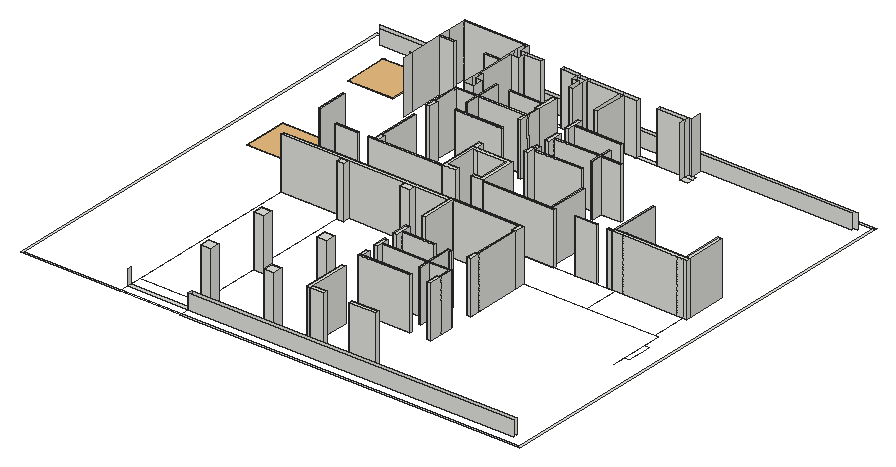
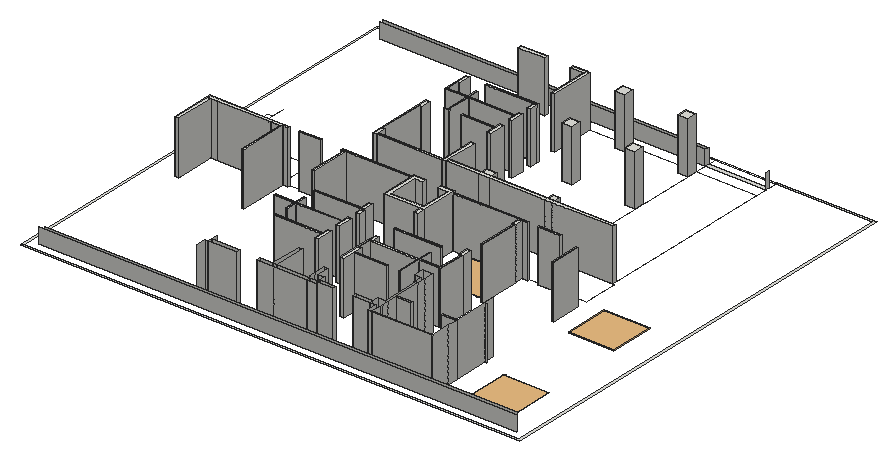
# SketchUp Ruby script. Lengths in inches.
U = 1.inch
M = Sketchup.active_model
def pt(a) = Geom::Point3d.new(a.map { |v| v * U })
def face(e, loops, mat)
  f = e.add_face(loops[0].map { |a| pt(a) })
  loops[1..].each { |l| e.add_face(l.map { |a| pt(a) }).erase! }
  f.material = f.back_material = mat if mat
  f
end
# faces: each face lists its corners as indices into pts; further lists are holes
def faces(e, pts, list, mat = nil) = list.each { |f| face(e, (f[0].is_a?(Array) ? f : [f]).map { |l| l.map { |i| pts[i] } }, mat) }
# xy, xz, yz: faces in a plane at the given z, y or x. An outline is a flat list of corners, or four numbers for a rectangle; further outlines are holes
def ring(l) = l.size == 4 ? [[l[0], l[1]], [l[2], l[1]], [l[2], l[3]], [l[0], l[3]]] : l.each_slice(2).to_a
def flat(e, list, mat, &to3) = list.each { |f| face(e, (f[0].is_a?(Array) ? f : [f]).map { |l| ring(l).map { |u, v| to3.(u, v) } }, mat) }
def xy(e, z, list, mat = nil) = flat(e, list, mat) { |x, y| [x, y, z] }
def xz(e, y, list, mat = nil) = flat(e, list, mat) { |x, z| [x, y, z] }
def yz(e, x, list, mat = nil) = flat(e, list, mat) { |y, z| [x, y, z] }
def lines(e, pts, list) = list.each { |a, b| e.add_line(pt(pts[a]), pt(pts[b])) }
# prism: a flat outline (further loops are holes) pulled along v
def prism(e, loops, v, mat = nil)
  f = face(e, loops, mat); d = Geom::Vector3d.new(v.map { |x| x * U })
  f.pushpull(f.normal.samedirection?(d) ? d.length : -d.length)
end
def box(e, o, s, mat = nil) = prism(e, [[o, [o[0] + s[0], o[1], o[2]], [o[0] + s[0], o[1] + s[1], o[2]], [o[0], o[1] + s[1], o[2]]]], [0, 0, s[2]], mat)
def at(x, y, z, deg = 0) = Geom::Transformation.translation(pt([x, y, z])) * Geom::Transformation.rotation(ORIGIN, Z_AXIS, deg.degrees)
def axes(o, x, y, z) = Geom::Transformation.new([*x, 0, *y, 0, *z, 0, *pt(o).to_a, 1])
def part(name) = M.definitions.add(name)
# library, detail: a bought-in or finely detailed component or shape, given as its bounding box
def library(name, o, s) = part(name).tap { |d| box(d.entities, o, s) }
def detail(e, o, s) = box(e.add_group.entities, o, s)
def put(e, d, t, mat = nil) = e.add_instance(d, t).tap { |i| i.material = mat if mat }
def group(e, t, mat = nil) = e.add_group.tap { |g| g.transformation = t; g.material = mat if mat }.entities
root = M.entities
c1 = library("BED",[-54,-53,-0.5],[108,106,1])
c2 = part("zw$FF1D")
put(c2.entities,c1,at(140.52,-153.67,0.04,-179.97))
put(c2.entities,c1,at(-181.99,-153.67,0.04,-179.97))
put(c2.entities,c1,at(-188.6,153.33,0.04,0.03))
box(root,[7152.21,596.5,1.375],[4.52,73.45,126])
box(root,[7210.71,572.45,1.375],[53.1,4.5,122.5625])
box(root,[7300.73,60,1.375],[24,24,122.5625])
box(root,[7300.73,217.5,1.375],[24,24,122.5625])
box(root,[7450.73,60,1.375],[24,24,122.5625])
box(root,[7450.73,217.5,1.375],[24,24,122.5625])
box(root,[7653.13,60,1.375],[63.82,9,122.5625])
xy(root,1.375,[[6920.46,0,7156.71,0,7156.71,4.5,6924.96,4.5,6924.96,1056.5,8106.96,1056.5,8106.96,1061,6920.46,1061],[7300.7,0,8102.46,4.5],[8102.46,0,8106.96,1056.5],[7156.71,24,7300.7,33],[7552.71,60,7561.71,165],
  [7561.71,60,7593.13,69],[7552.73,213,7676.4375,217.41],[7716.98,213,7725.96,241.45],[7552.73,217.41,7561.71,237],[7721.48,241.45,7725.96,271.5],
  [7669.71,247.5,7674.21,271.5],[7552.71,261,7561.71,292.1],[7561.71,271.5,7669.71,276],[7669.71,271.5,7674.21,276],[7674.21,271.5,7725.96,276],
  [7669.71,276,7674.21,331.02],[7552.71,316.1,7561.71,355],[7561.71,331,7638.96,335.5],[7716.98,331,7725.96,355],[7669.71,331.02,7674.21,331.5],
  [7674.21,331.02,7674.21,331.5,7669.71,331.5,7669.71,335.5,7680.96,335.5,7680.96,331.02],[7721.46,355,7725.96,464.5],[7552.7,403,7561.71,488.5],[7716.96,464.5,7725.98,488.5],[7300.71,464.55,7317.23,479.5],
  [7561.73,484.03,7716.96,488.5],[7450.73,488.5,7474.73,488.55],[7287.8125,572.5,7465.71,576.95],[7465.71,572.5,7465.71,662.5,7561.71,662.5,7561.71,572.5,7534.71,572.5,7534.71,581.5,7552.71,581.5,7552.71,653.5,7474.71,653.5,7474.71,581.5,7498.71,581.5,7498.71,572.5],[7561.71,572.5,7731.96,577],
  [7300.71,576.95,7309.73,596.85],[7719.96,577,7725.9375,670],[7300.71,596.85,7305.21,693.9375],[7465.71,662.5,7474.73,681.95],[7552.71,706,7561.71,730],
  [7561.71,725.5,7674.1875,730],[7300.73,730,7309.71,754],[7552.71,730,7561.71,745.14],[7353.21,749.45,7465.71,753.92],[7300.71,754,7305.23,818.45],
  [7669.71,760,7674.21,813.5],[7552.71,769.14,7561.71,804.6],[7561.71,784,7669.71,788.5],[7674.21,784,7721.46,788.5],[7465.71,795.95,7474.71,813.95],
  [7305.23,813.95,7353.21,818.45],[7357.71,813.95,7474.71,818.45],[7552.71,828.6,7561.71,867.45],[7300.71,843.5,7324.76,843.5,7324.76,867.5,7309.71,867.5,7309.71,886.95,7305.21,886.95,7305.21,977,7324.76,977,7324.76,1001,7309.7,1001,7309.7,1024.95,7300.71,1024.95,7300.71,952.95,7264.14,952.95,7264.14,948.45,7300.71,948.45],[7561.71,843.5,7674.1875,848],
  [7465.71,848,7474.71,900.43],[7552.71,915.5,7561.73,991.95],[7156.71,948.45,7193.27,952.95],[7708.01,977,7725.98,1001],[7324.76,991.95,7363.71,992],
  [7474.71,991.95,7552.71,992],[7552.71,991.95,7561.73,992],[7561.73,991.95,7592.49,992],[7324.76,992,7363.71,1001],[7450.7,992,7474.71,1001],
  [7474.71,992,7592.49,1001],[7592.49,992,7640.49,1001],[7640.49,992,7708.01,1001],[7411.71,1001,7450.7,1001.04],[7640.49,1001,7708.01,1001.04],
  [7156.71,1022.95,7300.71,1024.95]])
xy(root,4.8125,[[7552.71,706,7561.71,730]])
xy(root,123.9375,[[7552.71,60,7561.71,165],[7561.71,60,7593.13,69],[7552.73,213,7676.4375,217.41],[7716.98,213,7725.96,241.45],[7552.73,217.41,7561.71,237],
  [7721.48,241.45,7725.96,271.5],[7669.71,247.5,7674.21,271.5],[7552.71,261,7561.71,292.1],[7561.71,271.5,7669.71,276],[7669.71,271.5,7674.21,276],
  [7674.21,271.5,7725.96,276],[7669.71,276,7674.21,331.02],[7552.71,316.1,7561.71,355],[7561.71,331,7638.96,335.5],[7716.98,331,7725.96,355],
  [7674.21,331.02,7680.96,331.02,7680.96,335.5,7669.71,335.5,7669.71,331.5,7674.21,331.5],[7721.46,355,7725.96,464.5],[7552.7,403,7561.71,488.5],[7450.73,464.5,7474.73,479.5],[7716.96,464.5,7725.98,488.5],
  [7300.71,464.55,7317.23,479.5],[7156.71,479.5,7300.71,488.5],[7300.71,479.5,7317.23,488.5],[7317.23,479.5,7450.73,488.5],[7450.73,479.5,7474.73,488.5],
  [7474.73,479.5,7552.7,488.5],[7561.73,484.03,7716.96,488.5],[7287.8125,572.5,7465.71,576.95],[7561.71,572.5,7731.96,577],[7300.71,576.95,7309.73,596.85],
  [7719.96,577,7725.9375,670],[7300.71,596.85,7305.21,693.9375],[7561.71,725.5,7674.1875,730],[7552.71,730,7561.71,745.14],[7669.71,760,7674.21,813.5],
  [7552.71,769.14,7561.71,804.6],[7561.71,784,7669.71,788.5],[7674.21,784,7721.46,788.5],[7552.71,828.6,7561.71,867.45],[7561.71,843.5,7674.1875,848]])
xy(root,126,[[7353.21,749.45,7465.71,753.92]])
xy(root,127.375,[[7465.71,572.5,7498.71,572.5,7498.71,581.5,7474.71,581.5,7474.71,653.5,7552.71,653.5,7552.71,581.5,7534.71,581.5,7534.71,572.5,7561.71,572.5,7561.71,662.5,7465.71,662.5],[7465.71,662.5,7474.73,681.95],[7552.71,706,7561.71,730],[7300.73,730,7309.71,754],[7353.21,749.45,7465.71,753.92],
  [7300.71,754,7305.23,818.45],[7353.21,783.95,7357.71,871.95],[7465.71,795.95,7474.7,813.95],[7305.23,813.95,7353.21,818.45],[7357.71,813.95,7474.7,813.95,7474.71,818.45,7357.71,818.45],
  [7470.21,818.45,7474.71,847.95],[7465.71,848,7474.71,900.43],[7387.71,867.45,7465.71,871.95]])
xz(root,24,[[7300.7,1.375,8073.98,37.375]])
xz(root,33,[[7300.7,1.375,8073.98,37.375]])
xz(root,60,[[7552.71,1.375,7561.71,123.9375],[7561.71,1.375,7593.13,123.9375]])
xz(root,69,[[7561.71,1.375,7593.13,123.9375]])
xz(root,165,[[7552.71,1.375,7561.71,123.9375]])
xz(root,213,[[7552.73,1.375,7676.4375,123.9375],[7716.98,1.375,7725.96,123.9375]])
xz(root,217.41,[[7552.73,1.375,7561.71,123.9375],[7561.71,1.375,7676.4375,123.9375]])
xz(root,237,[[7552.73,1.375,7561.71,123.9375]])
xz(root,241.45,[[7716.98,1.375,7721.48,123.9375],[7721.48,1.375,7725.96,123.9375]])
xz(root,247.5,[[7669.71,1.375,7674.21,123.9375]])
xz(root,261,[[7552.71,1.375,7561.71,123.9375]])
xz(root,271.5,[[7561.71,1.375,7669.71,123.9375],[7669.71,1.375,7674.21,123.9375],[7674.21,1.375,7721.48,123.9375],[7721.48,1.375,7725.96,123.9375]])
xz(root,276,[[7561.71,1.375,7669.71,123.9375],[7669.71,1.375,7674.21,123.9375],[7674.21,1.375,7725.96,123.9375]])
xz(root,292.1,[[7552.71,1.375,7561.71,123.9375]])
xz(root,316.1,[[7552.71,1.375,7561.71,123.9375]])
xz(root,331,[[7561.71,1.375,7638.96,123.9375],[7716.98,1.375,7725.96,123.9375]])
xz(root,331.02,[[7669.71,1.375,7674.21,123.9375],[7674.21,1.375,7680.96,123.9375]])
xz(root,331.5,[[7669.71,1.375,7674.21,123.9375]])
xz(root,335.5,[[7561.71,1.375,7638.96,123.9375],[7669.71,1.375,7680.96,123.9375]])
xz(root,355,[[7552.71,1.375,7561.71,123.9375],[7716.98,1.375,7721.46,123.9375],[7721.46,1.375,7725.96,123.9375]])
xz(root,403,[[7552.7,1.375,7561.71,123.9375]])
xz(root,464.5,[[7450.73,1.375,7474.73,123.9375],[7716.96,1.375,7721.46,123.9375],[7721.46,1.375,7725.96,123.9375],[7725.96,1.375,7725.98,123.9375]])
xz(root,464.55,[[7300.71,1.375,7317.23,123.9375]])
xz(root,479.5,[[7156.71,1.375,7300.71,123.9375],[7300.71,1.375,7317.23,123.9375],[7317.23,1.375,7450.73,123.9375],[7474.73,1.375,7552.7,123.9375]])
xz(root,484.03,[[7561.73,1.375,7716.96,123.9375]])
xz(root,488.5,[[7156.71,1.375,7300.71,123.9375],[7300.71,1.375,7317.23,123.9375],[7317.23,1.375,7450.73,123.9375],[7450.73,1.375,7474.73,123.9375],[7474.73,1.375,7552.7,123.9375],
  [7552.7,1.375,7561.71,123.9375],[7561.73,1.375,7716.96,123.9375],[7716.96,1.375,7725.98,123.9375]])
xz(root,572.5,[[7287.8125,1.375,7465.71,123.9375],[7465.71,1.375,7498.71,127.375],[7534.71,1.375,7561.71,127.375],[7561.71,1.375,7731.96,123.9375]])
xz(root,576.95,[[7287.8125,1.375,7300.71,123.9375],[7300.71,1.375,7309.73,123.9375],[7309.73,1.375,7465.71,123.9375]])
xz(root,577,[[7561.71,1.375,7719.96,123.9375],[7719.96,1.375,7725.9375,123.9375],[7725.9375,1.375,7731.96,123.9375]])
xz(root,581.5,[[7474.71,1.375,7498.71,127.375],[7534.71,1.375,7552.71,127.375]])
xz(root,596.85,[[7300.71,1.375,7305.21,123.9375],[7305.21,1.375,7309.73,123.9375]])
xz(root,653.5,[[7474.71,1.375,7481.96,127.375],[7481.96,1.375,7545.45,127.375],[7545.45,1.375,7552.71,127.375]])
xz(root,662.5,[[7465.71,1.375,7474.73,127.375],[7474.73,1.375,7561.71,127.375]])
xz(root,670,[[7719.96,1.375,7725.9375,123.9375]])
xz(root,681.95,[[7465.71,1.375,7474.73,127.375]])
xz(root,693.9375,[[7300.71,1.375,7305.21,123.9375]])
xz(root,706,[[7552.71,1.375,7561.71,4.8125],[7552.71,4.8125,7561.71,127.375]])
xz(root,725.5,[[7561.71,1.375,7674.1875,123.9375]])
xz(root,730,[[7300.73,1.375,7309.71,127.375],[7552.71,1.375,7561.71,4.8125],[7561.71,1.375,7674.1875,123.9375],[7552.71,4.8125,7561.71,123.9375],[7552.71,123.9375,7561.71,127.375]])
xz(root,745.14,[[7552.71,1.375,7561.71,123.9375]])
xz(root,749.45,[[7353.21,1.375,7465.71,126],[7353.21,126,7465.71,127.375]])
xz(root,753.92,[[7353.21,1.375,7465.71,126],[7353.21,126,7465.71,127.375]])
xz(root,754,[[7300.71,1.375,7300.73,127.375],[7300.73,1.375,7305.23,127.375],[7305.23,1.375,7309.71,127.375]])
xz(root,760,[[7669.71,1.375,7674.21,123.9375]])
xz(root,769.14,[[7552.71,1.375,7561.71,123.9375]])
xz(root,783.95,[[7353.21,1.375,7357.71,127.375]])
xz(root,784,[[7561.71,1.375,7669.71,123.9375],[7674.21,1.375,7721.46,123.9375]])
xz(root,788.5,[[7561.71,1.375,7669.71,123.9375],[7674.21,1.375,7721.46,123.9375]])
xz(root,795.95,[[7465.71,1.375,7474.71,1.375,7474.7,127.375,7465.71,127.375]])
xz(root,804.6,[[7552.71,1.375,7561.71,123.9375]])
xz(root,813.5,[[7669.71,1.375,7674.21,123.9375]])
xz(root,813.95,[[7305.23,1.375,7353.21,127.375],[7357.71,1.375,7465.71,127.375],[7465.71,1.375,7465.71,127.375,7474.7,127.375,7474.71,1.375]])
xz(root,818.45,[[7300.71,1.375,7305.23,127.375],[7305.23,1.375,7353.21,127.375],[7357.71,1.375,7470.21,127.375],[7470.21,1.375,7474.71,127.375]])
xz(root,828.6,[[7552.71,1.375,7561.71,123.9375]])
xz(root,843.5,[[7300.71,1.375,7324.76,127.375],[7561.71,1.375,7674.1875,123.9375]])
xz(root,847.95,[[7470.21,1.375,7474.71,127.375]])
xz(root,848,[[7465.71,1.375,7474.71,127.375],[7561.71,1.375,7674.1875,123.9375]])
xz(root,867.45,[[7152.23,1.375,7156.71,127.375],[7387.71,1.375,7465.71,127.375],[7552.71,1.375,7561.71,123.9375]])
xz(root,867.5,[[7309.71,1.375,7324.76,127.375]])
xz(root,871.95,[[7353.21,1.375,7357.71,127.375],[7387.71,1.375,7465.71,127.375]])
xz(root,886.95,[[7305.21,1.375,7309.71,127.375]])
xz(root,900.43,[[7465.71,1.375,7474.71,127.375]])
xz(root,915.5,[[7552.71,1.375,7561.73,123.9375]])
xz(root,948.43,[[7465.71,1.375,7474.71,127.375]])
xz(root,948.45,[[7156.71,1.375,7193.27,127.375],[7264.14,1.375,7300.71,127.375]])
xz(root,952.95,[[7156.71,1.375,7193.27,127.375],[7264.14,1.375,7300.71,127.375]])
xz(root,976.95,[[7450.7,1.375,7465.71,127.375]])
xz(root,977,[[7305.21,1.375,7324.76,127.375]])
xz(root,991.95,[[7552.71,1.375,7561.73,123.9375]])
xz(root,992,[[7324.76,1.375,7363.71,127.375],[7411.71,1.375,7450.7,127.375],[7450.7,1.375,7474.71,123.9375],[7474.71,1.375,7552.71,123.9375],[7552.71,1.375,7561.73,123.9375],
  [7561.73,1.375,7592.49,123.9375],[7640.49,1.375,7708.01,123.9375]])
xz(root,1001,[[7309.7,1.375,7324.76,127.375],[7324.76,1.375,7363.71,127.375],[7411.71,1.375,7450.7,127.375],[7450.7,1.375,7474.71,123.9375],[7474.71,1.375,7552.71,123.9375],
  [7552.71,1.375,7592.49,123.9375],[7640.49,1.375,7708.01,123.9375],[7708.01,1.375,7716.96,123.9375]])
xz(root,1022.95,[[7156.71,1.375,7300.71,127.375]])
xz(root,1024.95,[[7156.71,1.375,7300.71,127.375],[7300.71,1.375,7309.7,127.375]])
xz(root,1028,[[6953.48,1.375,8073.98,37.375]])
xz(root,1037,[[6944.48,1.375,8082.98,37.375]])
yz(root,7156.71,[[24,1.375,33,37.375],[479.5,1.375,488.5,123.9375],[843.45,1.375,867.45,127.375],[867.45,1.375,948.45,127.375],[952.95,1.375,976.95,127.375],
  [976.95,1.375,1022.95,127.375],[1022.95,1.375,1024.95,127.375]])
yz(root,7193.27,[[948.45,1.375,952.95,127.375]])
yz(root,7264.14,[[948.45,1.375,952.95,127.375]])
yz(root,7287.8125,[[572.5,1.375,576.95,123.9375]])
yz(root,7300.7,[[24,1.375,33,37.375]])
yz(root,7300.71,[[464.55,1.375,479.5,123.9375],[576.95,1.375,596.85,123.9375],[596.85,1.375,693.9375,123.9375],[754,1.375,818.45,127.375],[843.5,1.375,867.5,127.375],
  [867.5,1.375,886.95,127.375],[886.95,1.375,948.45,127.375],[952.95,1.375,977,127.375],[977,1.375,992,127.375],[992,1.375,1001,127.375],
  [1001,1.375,1022.95,127.375],[1022.95,1.375,1024.95,127.375]])
yz(root,7300.73,[[730,1.375,754,127.375]])
yz(root,7305.21,[[596.85,1.375,693.9375,123.9375],[886.95,1.375,977,127.375]])
yz(root,7305.23,[[754,1.375,813.95,127.375],[813.95,1.375,818.45,127.375]])
yz(root,7309.7,[[1001,1.375,1024.95,127.375]])
yz(root,7309.71,[[730,1.375,754,127.375],[867.5,1.375,886.95,127.375]])
yz(root,7309.73,[[576.95,1.375,596.85,123.9375]])
yz(root,7317.23,[[464.55,1.375,479.5,123.9375]])
yz(root,7324.76,[[843.5,1.375,867.5,127.375],[977,1.375,992,127.375],[992,1.375,1001,127.375]])
yz(root,7353.21,[[749.45,1.375,753.92,126],[783.95,1.375,813.95,127.375],[813.95,1.375,818.45,127.375],[818.45,1.375,871.95,127.375],[749.45,126,753.92,127.375]])
yz(root,7357.71,[[783.95,1.375,813.95,127.375],[813.95,1.375,818.45,127.375],[818.45,1.375,871.95,127.375]])
yz(root,7363.71,[[992,1.375,1001,127.375]])
yz(root,7387.71,[[867.45,1.375,871.95,127.375]])
yz(root,7411.71,[[992,1.375,1001,127.375]])
yz(root,7450.7,[[976.95,1.375,992,127.375],[992,1.375,1001,123.9375]])
yz(root,7450.73,[[464.5,1.375,479.5,123.9375]])
yz(root,7465.71,[[572.5,1.375,576.95,123.9375],[576.95,1.375,662.5,127.375],[662.5,1.375,681.95,127.375],[749.45,1.375,753.92,126],[795.95,1.375,813.95,127.375],
  [848,1.375,867.45,127.375],[871.95,1.375,900.43,127.375],[948.43,1.375,976.95,127.375],[572.5,123.9375,576.95,127.375],[749.45,126,753.92,127.375]])
yz(root,7470.21,[[818.45,1.375,847.95,127.375]])
yz(root,7474.71,[[581.5,1.375,653.5,127.375],[818.45,1.375,847.95,127.375],[848,1.375,900.43,127.375],[948.43,1.375,976.95,127.375],[976.95,1.375,991.95,127.375],
  [991.95,1.375,992,127.375],[992,1.375,1001,123.9375]])
yz(root,7474.73,[[464.5,1.375,479.5,123.9375],[662.5,1.375,681.95,127.375]])
yz(root,7498.71,[[572.5,1.375,581.5,127.375]])
yz(root,7534.71,[[572.5,1.375,581.5,127.375]])
yz(root,7552.7,[[403,1.375,479.5,123.9375],[479.5,1.375,488.5,123.9375]])
yz(root,7552.71,[[60,1.375,165,123.9375],[261,1.375,292.1,123.9375],[316.1,1.375,355,123.9375],[581.5,1.375,653.5,127.375],[706,1.375,730,4.8125],
  [730,1.375,745.14,123.9375],[769.14,1.375,804.6,123.9375],[828.6,1.375,867.45,123.9375],[915.5,1.375,991.95,123.9375],[706,4.8125,730,127.375]])
yz(root,7552.73,[[213,1.375,217.41,123.9375],[217.41,1.375,237,123.9375]])
yz(root,7561.71,[[60,1.375,69,123.9375],[69,1.375,165,123.9375],[217.41,1.375,237,123.9375],[261,1.375,271.5,123.9375],[271.5,1.375,276,123.9375],
  [276,1.375,292.1,123.9375],[316.1,1.375,331,123.9375],[331,1.375,335.5,123.9375],[335.5,1.375,355,123.9375],[403,1.375,484.03,123.9375],
  [484.03,1.375,488.5,123.9375],[572.5,1.375,577,123.9375],[577,1.375,662.5,127.375],[706,1.375,725.5,4.8125],[725.5,1.375,730,4.8125],
  [730,1.375,745.14,123.9375],[769.14,1.375,784,123.9375],[784,1.375,788.5,123.9375],[788.5,1.375,804.6,123.9375],[828.6,1.375,843.5,123.9375],
  [843.5,1.375,848,123.9375],[848,1.375,867.45,123.9375],[706,4.8125,725.5,127.375],[725.5,4.8125,730,123.9375],[572.5,123.9375,577,127.375],
  [725.5,123.9375,730,127.375]])
yz(root,7561.73,[[484.03,1.375,488.5,123.9375],[915.5,1.375,991.95,123.9375]])
yz(root,7592.49,[[992,1.375,1001,123.9375]])
yz(root,7593.13,[[60,1.375,69,123.9375]])
yz(root,7638.96,[[331,1.375,335.5,123.9375]])
yz(root,7640.49,[[992,1.375,1001,123.9375]])
yz(root,7669.71,[[247.5,1.375,271.5,123.9375],[271.5,1.375,276,123.9375],[276,1.375,331.02,123.9375],[331.5,1.375,335.5,123.9375],[760,1.375,784,123.9375],
  [784,1.375,788.5,123.9375],[788.5,1.375,813.5,123.9375]])
yz(root,7674.1875,[[725.5,1.375,730,123.9375],[843.5,1.375,848,123.9375]])
yz(root,7674.21,[[247.5,1.375,271.5,123.9375],[271.5,1.375,276,123.9375],[276,1.375,331.02,123.9375],[331.02,1.375,331.5,123.9375],[760,1.375,784,123.9375],
  [784,1.375,788.5,123.9375],[788.5,1.375,813.5,123.9375]])
yz(root,7676.4375,[[213,1.375,217.41,123.9375]])
yz(root,7680.96,[[331.02,1.375,335.5,123.9375]])
yz(root,7708.01,[[977,1.375,992,123.9375],[992,1.375,1001,123.9375]])
yz(root,7716.96,[[464.5,1.375,484.03,123.9375],[484.03,1.375,488.5,123.9375],[1001,1.375,1025,123.9375]])
yz(root,7716.98,[[213,1.375,241.45,123.9375],[331,1.375,355,123.9375]])
yz(root,7719.96,[[577,1.375,670,123.9375]])
yz(root,7721.46,[[355,1.375,464.5,123.9375],[784,1.375,788.5,123.9375]])
yz(root,7721.48,[[241.45,1.375,271.5,123.9375]])
yz(root,7725.9375,[[577,1.375,670,123.9375]])
yz(root,7725.96,[[213,1.375,241.45,123.9375],[241.45,1.375,271.5,123.9375],[271.5,1.375,276,123.9375],[331,1.375,355,123.9375],[355,1.375,464.5,123.9375]])
yz(root,7725.98,[[464.5,1.375,488.5,123.9375]])
yz(root,7731.96,[[572.5,1.375,577,123.9375]])
p = [[7474.71,795.95,1.375],[7474.71,813.95,1.375],[7474.7,813.95,127.375],[7474.7,795.95,127.375],[7474.71,818.45,1.375],[7474.71,818.45,127.375],
  [7540.91,642.62,1.375],[7544.84,646.24,1.375],[7486.5,642.62,1.375],[7513.71,617.5,1.375],[7481.96,642.62,1.375],[7545.45,646.8,1.375],
  [7545.45,653.5,1.375],[7483.93,590.01,1.375],[7481.96,646.8,1.375],[7482.57,646.24,1.375],[7481.96,646.24,1.375],[7228.7,0,1.375],
  [7156.71,0,1.375],[7543.48,590.01,1.375],[7300.7,24,1.375],[7300.7,4.5,1.375],[7156.71,33,1.375],[7156.71,60,1.375],
  [7156.71,4.5,1.375],[7156.71,24,1.375],[7300.7,60,1.375],[7300.7,33,1.375],[7300.7,0,1.375],[7300.73,60,1.375],
  [7552.71,653.5,1.375],[7545.45,642.62,1.375],[7498.71,581.5,1.375],[7534.71,581.5,1.375],[7708.01,992,1.375],[7725.96,992,1.375],
  [7156.71,455.83,1.375],[7156.71,479.5,1.375],[7474.71,653.5,1.375],[7545.45,590.01,1.375],[7474.71,581.5,1.375],[7481.96,590.01,1.375],
  [7481.96,653.5,1.375],[7300.71,437.9,1.375],[7545.45,646.24,1.375],[7498.71,572.5,1.375],[7534.71,572.5,1.375],[7561.71,484.03,1.375],
  [7561.73,484.03,1.375],[7552.71,581.5,1.375],[7324.73,60,1.375],[7552.71,60,1.375],[7300.71,464.55,1.375],[7363.71,992,1.375],
  [7411.71,992,1.375],[7363.71,1001,1.375],[7411.71,1001,1.375]]
faces(root,p,[[0,1,2,3],[1,4,5,2]])
lines(root,p,[[6,7],[8,9],[8,10],[11,12],[13,9],[14,15],[14,16],[6,8],[17,18],[13,19],[15,7],[9,19],
  [15,8],[9,6],[20,21],[22,23],[24,21],[24,25],[23,26],[26,27],[28,17],[26,29],[11,30],[31,6],
  [32,33],[34,35],[36,37],[38,14],[39,31],[7,11],[40,13],[10,41],[42,14],[23,36],[43,26],[16,15],
  [7,44],[19,39],[45,46],[41,13],[47,48],[44,11],[19,49],[50,51],[52,43],[53,54],[55,56]])
put(root,c2,at(7232.87,784.63,1.83))
g1 = group(root,at(7152.21,355,1.375))
box(g1,[627.75,217.45,0],[53.11,4.55,126])
xy(g1,0,[[717.77,217.45,741.75,226.5],[870.75,217.45,870.75,226.45,741.75,226.45,741.75,226.5,894.75,226.5,894.75,217.45],[717.64,226.5,722.25,338.66],[885.75,226.5,894.75,322.5]])
xy(g1,126,[[717.77,217.45,741.75,226.5],[741.75,217.45,870.75,226.45],[870.75,217.45,894.75,217.45,894.75,226.5,741.75,226.5,741.75,226.45,870.75,226.45],[704.86,217.5,717.77,221.95],[717.64,226.5,722.25,338.66],
  [885.75,226.5,894.75,322.5]])
xz(g1,217.45,[[717.77,0,741.75,126],[741.75,0,870.75,126],[870.75,0,885.75,126],[885.75,0,894.75,126]])
xz(g1,217.5,[[704.86,0,717.77,126]])
xz(g1,221.95,[[704.86,0,717.77,126]])
xz(g1,226.5,[[717.64,0,717.77,126],[717.77,0,722.25,126],[722.25,0,741.75,126],[741.75,0,885.75,126],[885.75,0,894.75,126]])
xz(g1,322.5,[[885.75,0,894.75,126]])
xz(g1,338.66,[[717.64,0,722.25,126]])
yz(g1,704.86,[[217.5,0,221.95,126]])
yz(g1,717.64,[[226.5,0,338.66,126]])
yz(g1,717.77,[[217.45,0,217.5,126],[221.95,0,226.5,126]])
yz(g1,722.25,[[226.5,0,338.66,126]])
yz(g1,741.75,[[226.45,0,226.5,126]])
yz(g1,885.75,[[226.5,0,322.5,126]])
yz(g1,894.75,[[217.45,0,226.5,126],[226.5,0,322.5,126]])
p = [[4.5,133.5,0],[400.5,133.5,0],[723.75,133.5,0],[885.75,133.5,0],[885.75,217.45,0],[894.78,91.46,0],
  [894.78,31.46,0],[894.75,31.46,0],[148.5,124.5,0],[4.5,124.5,0],[906.75,91.46,0],[894.78,0,0],
  [894.78,133.5,0],[313.5,217.45,0],[627.75,217.45,0],[894.75,91.46,0],[885.75,226.45,0],[906.75,31.46,0],
  [0,133.5,0],[723.75,217.45,0],[0,217.45,0],[680.86,217.45,0],[717.77,217.45,0],[870.75,226.45,0],
  [870.75,226.45,126]]
lines(g1,p,[[0,1],[2,3],[4,3],[5,6],[6,7],[8,9],[5,10],[6,11],[1,2],[3,12],[13,14],[15,5],
  [16,4],[12,5],[10,17],[17,6],[18,0],[2,19],[20,18],[19,20],[21,22],[23,24]])
